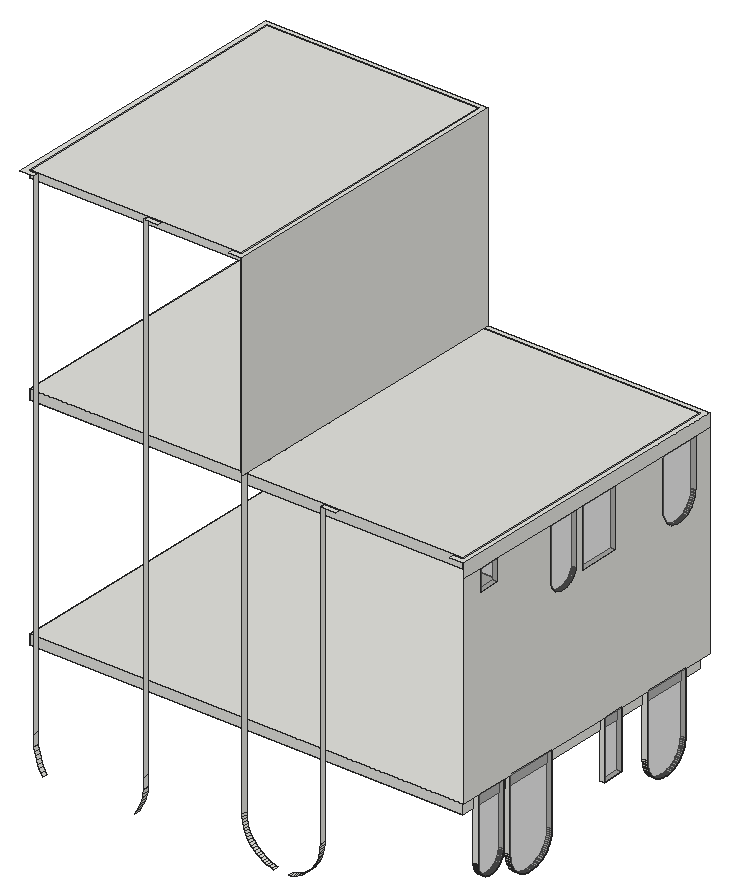
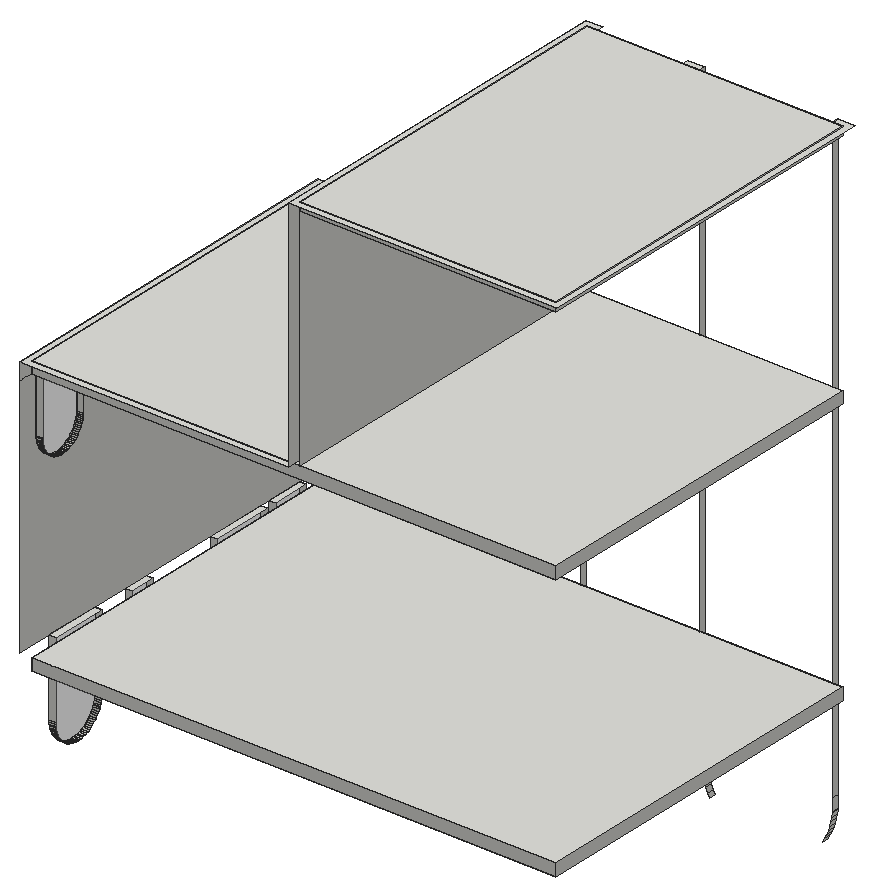
# SketchUp Ruby script. Lengths in inches.
U = 1.inch
M = Sketchup.active_model
def pt(a) = Geom::Point3d.new(a.map { |v| v * U })
def face(e, loops, mat)
  f = e.add_face(loops[0].map { |a| pt(a) })
  loops[1..].each { |l| e.add_face(l.map { |a| pt(a) }).erase! }
  f.material = f.back_material = mat if mat
  f
end
# faces: each face lists its corners as indices into pts; further lists are holes
def faces(e, pts, list, mat = nil) = list.each { |f| face(e, (f[0].is_a?(Array) ? f : [f]).map { |l| l.map { |i| pts[i] } }, mat) }
# xy, xz, yz: faces in a plane at the given z, y or x. An outline is a flat list of corners, or four numbers for a rectangle; further outlines are holes
def ring(l) = l.size == 4 ? [[l[0], l[1]], [l[2], l[1]], [l[2], l[3]], [l[0], l[3]]] : l.each_slice(2).to_a
def flat(e, list, mat, &to3) = list.each { |f| face(e, (f[0].is_a?(Array) ? f : [f]).map { |l| ring(l).map { |u, v| to3.(u, v) } }, mat) }
def xy(e, z, list, mat = nil) = flat(e, list, mat) { |x, y| [x, y, z] }
def xz(e, y, list, mat = nil) = flat(e, list, mat) { |x, z| [x, y, z] }
def yz(e, x, list, mat = nil) = flat(e, list, mat) { |y, z| [x, y, z] }
def lines(e, pts, list) = list.each { |a, b| e.add_line(pt(pts[a]), pt(pts[b])) }
# prism: a flat outline (further loops are holes) pulled along v
def prism(e, loops, v, mat = nil)
  f = face(e, loops, mat); d = Geom::Vector3d.new(v.map { |x| x * U })
  f.pushpull(f.normal.samedirection?(d) ? d.length : -d.length)
end
def box(e, o, s, mat = nil) = prism(e, [[o, [o[0] + s[0], o[1], o[2]], [o[0] + s[0], o[1] + s[1], o[2]], [o[0], o[1] + s[1], o[2]]]], [0, 0, s[2]], mat)
def at(x, y, z, deg = 0) = Geom::Transformation.translation(pt([x, y, z])) * Geom::Transformation.rotation(ORIGIN, Z_AXIS, deg.degrees)
def axes(o, x, y, z) = Geom::Transformation.new([*x, 0, *y, 0, *z, 0, *pt(o).to_a, 1])
def part(name) = M.definitions.add(name)
# library, detail: a bought-in or finely detailed component or shape, given as its bounding box
def library(name, o, s) = part(name).tap { |d| box(d.entities, o, s) }
def detail(e, o, s) = box(e.add_group.entities, o, s)
def put(e, d, t, mat = nil) = e.add_instance(d, t).tap { |i| i.material = mat if mat }
def group(e, t, mat = nil) = e.add_group.tap { |g| g.transformation = t; g.material = mat if mat }.entities
root = M.entities
M.materials.add("[Translucent Glass Gray]").color = [128, 128, 128]
M.materials["[Translucent Glass Gray]"].alpha = 0.5
c1 = part("Group\#2")
box(c1.entities,[0,0,0],[753.47,516,17])
box(root,[1479.625,496.08,1382],[368.1,516,12])
xy(root,576.55,[[2233.1,793.72,2242.1,831.72]])
xy(root,678.55,[[2233.1,518.83,2242.1,573.83],[2233.1,588.16,2242.1,679.32],[2233.1,793.72,2242.1,831.72],[2233.1,886.32,2242.1,969.32]])
xy(root,928.39,[[2233.1,745.0625,2242.1,818.41]])
xy(root,991.35,[[2233.1,523.83,2242.1,561.87]])
xy(root,1029.2,[[2233.1,523.83,2242.1,561.87],[2233.1,675.625,2242.1,733.55],[2233.1,745.0625,2242.1,818.41],[2233.1,919.74,2242.1,992.74]])
xy(root,1054,[[2218.1,487.08,2242.1,487.08,2242.1,1021.08,1856.72,1021.08,1856.72,1012.08,2233.1,1012.08,2233.1,496.08,2218.1,496.08],[1992.57,487.08,2019.16,496.08],[1847.72,496.08,1856.72,1012.08]])
xy(root,1394,[[1470.625,487.08,1494.625,487.08,1494.625,496.08,1479.625,496.08,1479.625,1012.08,1847.72,1012.08,1847.72,496.08,1832.72,496.08,1832.72,487.08,1856.72,487.08,1856.72,1021.08,1470.625,1021.08],[1685.42,487.08,1709.42,496.08]])
xz(root,487.08,[[1494.625,505.5,1494.625,523.51,1494.22,517.14,1494.25,510.75],[1685.42,505.5,1685.79,510.75,1685.82,517.14,1685.42,523.51]])
xz(root,518.83,[[2233.1,569.55,2242.1,678.55]])
xz(root,523.83,[[2233.1,991.35,2242.1,1029.2]])
xz(root,561.87,[[2233.1,991.35,2242.1,1029.2]])
xz(root,573.83,[[2233.1,569.55,2242.1,678.55]])
xz(root,588.16,[[2233.1,554.92,2242.1,678.55]])
xz(root,675.625,[[2233.1,938.71,2242.1,1029.2]])
xz(root,679.32,[[2233.1,554.92,2242.1,678.55]])
xz(root,733.55,[[2233.1,938.71,2242.1,1029.2]])
xz(root,745.0625,[[2233.1,928.39,2242.1,1029.2]])
xz(root,793.72,[[2233.1,576.55,2242.1,678.55]])
xz(root,818.41,[[2233.1,928.39,2242.1,1029.2]])
xz(root,831.72,[[2233.1,576.55,2242.1,678.55]])
xz(root,886.32,[[2233.1,569.55,2242.1,678.55]])
xz(root,919.74,[[2233.1,946.2,2242.1,1029.2]])
xz(root,969.32,[[2233.1,569.55,2242.1,678.55]])
xz(root,992.74,[[2233.1,946.2,2242.1,1029.2]])
yz(root,1494.625,[[487.08,505.5,496.08,523.51],[487.08,523.51,496.08,1394]])
yz(root,1685.42,[[487.08,505.5,496.08,523.51],[487.08,523.51,496.08,1394]])
yz(root,1847.72,[[496.08,1054,1012.08,1394]])
yz(root,1856.72,[[487.08,527,496.08,1054],[487.08,1054,1021.08,1394]])
yz(root,1992.57,[[487.08,527,496.08,1054]])
yz(root,2242.1,[[487.08,678.55,1021.08,678.55,1021.08,1029.2,992.74,1029.2,992.74,946.2,992.67,943.9,992.46,941.62,992.1,939.36,991.6,937.12,990.96,934.92,990.18,932.76,989.27,930.66,988.23,928.61,987.0625,926.64,985.77,924.74,984.37,922.93,982.85,921.21,981.23,919.59,979.51,918.07,977.7,916.67,975.8,915.38,973.83,914.21,971.78,913.17,969.68,912.26,967.52,911.48,965.32,910.84,963.08,910.34,960.82,909.98,958.54,909.77,956.24,909.7,953.95,909.77,951.67,909.98,949.4,910.34,947.17,910.84,944.96,911.48,942.81,912.26,940.7,913.17,938.66,914.21,936.6875,915.38,934.79,916.67,932.98,918.07,931.26,919.59,929.64,921.21,928.12,922.93,926.71,924.74,925.43,926.64,924.26,928.61,923.22,930.66,922.31,932.76,921.53,934.92,920.89,937.12,920.39,939.36,920.03,941.62,919.82,943.9,919.74,946.2,919.74,1029.2,818.41,1029.2,818.41,928.39,745.0625,928.39,745.0625,1029.2,733.55,1029.2,733.55,938.71,733.14,937.17,732.65,935.66,732.08,934.17,731.43,932.72,730.7,931.3,729.9,929.92,729.03,928.59,728.08,927.31,727.07,926.08,726,924.9,724.86,923.79,723.67,922.73,722.42,921.75,721.12,920.83,719.77,919.98,718.375,919.2,716.95,918.5,715.48,917.88,713.98,917.34,712.46,916.875,710.91,916.5,709.35,916.2,707.77,915.99,706.18,915.86,704.59,915.82,703,915.86,701.41,915.99,699.83,916.2,698.27,916.5,696.72,916.875,695.19,917.34,693.7,917.88,692.23,918.5,690.8,919.2,689.41,919.98,688.0625,920.83,686.76,921.75,685.51,922.73,684.32,923.79,683.18,924.9,682.1,926.08,681.09,927.31,680.15,928.59,679.28,929.92,678.47,931.3,677.75,932.72,677.1,934.17,676.53,935.66,676.04,937.17,675.625,938.71,675.625,1029.2,561.87,1029.2,561.87,991.35,523.83,991.35,523.83,1029.2,487.08,1029.2],[487.08,1029.2,1021.08,1054]])
yz(root,2242.1,[[633.74,509.34,636.6,509.43,639.45,509.7,642.28,510.15,645.07,510.78,647.82,511.57,650.51,512.54,653.14,513.68,655.69,514.98,658.16,516.4375,660.53,518.05,662.79,519.8,664.9375,521.7,666.96,523.72,668.86,525.87,670.61,528.13,672.22,530.5,673.68,532.96,674.98,535.52,676.11,538.14,677.08,540.84,677.88,543.59,678.51,546.38,678.96,549.21,679.23,552.0625,679.32,554.92,679.32,678.55,588.16,678.55,588.16,554.92,588.25,552.0625,588.52,549.21,588.96,546.38,589.59,543.59,590.39,540.84,591.36,538.14,592.49,535.52,593.79,532.96,595.25,530.5,596.86,528.13,598.62,525.87,600.51,523.72,602.53,521.7,604.68,519.8,606.94,518.05,609.3125,516.4375,611.78,514.98,614.33,513.68,616.96,512.54,619.65,511.57,622.4,510.78,625.19,510.15,628.02,509.7,630.875,509.43],[927.82,528.05,930.42,528.14,933.02,528.38,935.59,528.79,938.14,529.36,940.64,530.09,943.09,530.97,945.49,532,947.81,533.1875,950.05,534.51,952.21,535.98,954.27,537.58,956.22,539.3,958.07,541.15,959.79,543.1,961.39,545.16,962.86,547.32,964.18,549.5625,965.37,551.88,966.4,554.28,966.63,554.92,967.28,556.73,968.01,559.23,968.58,561.78,968.99,564.35,969.23,566.95,969.32,569.55,969.32,678.55,886.32,678.55,886.32,569.55,886.4,566.95,886.64,564.35,887.05,561.78,887.62,559.23,888.35,556.73,889,554.92,889.23,554.28,890.27,551.88,891.45,549.5625,892.78,547.32,894.24,545.16,895.84,543.1,897.5625,541.15,899.41,539.3,901.36,537.58,903.42,535.98,905.58,534.51,907.82,533.1875,910.15,532,912.54,530.97,914.99,530.09,917.5,529.36,920.04,528.79,922.61,528.38,925.21,528.14],[546.33,542.05,548.05,542.11,549.77,542.27,551.48,542.54,553.17,542.92,554.82,543.4,556.45,543.99,558.04,544.67,559.58,545.46,561.0625,546.33,562.49,547.31,563.86,548.36,565.15,549.51,566.375,550.73,567.52,552.02,568.57,553.39,569.55,554.82,569.61,554.92,570.43,556.31,571.21,557.84,571.9,559.43,572.48,561.06,572.96,562.71,573.34,564.4,573.61,566.11,573.77,567.83,573.83,569.55,573.83,678.55,518.83,678.55,518.83,569.55,518.88,567.83,519.04,566.11,519.3125,564.4,519.69,562.71,520.17,561.06,520.76,559.43,521.44,557.84,522.23,556.31,523.05,554.92,523.11,554.82,524.08,553.39,525.14,552.02,526.28,550.73,527.5,549.51,528.8,548.36,530.16,547.31,531.59,546.33,533.08,545.46,534.62,544.67,536.2,543.99,537.83,543.4,539.49,542.92,541.17,542.54,542.88,542.27,544.6,542.11],[793.72,576.55,831.72,678.55],[956.24,909.7,958.54,909.77,960.82,909.98,963.08,910.34,965.32,910.84,967.52,911.48,969.68,912.26,971.78,913.17,973.83,914.21,975.8,915.38,977.7,916.67,979.51,918.07,981.23,919.59,982.85,921.21,984.37,922.93,985.77,924.74,987.0625,926.64,988.23,928.61,989.27,930.66,990.18,932.76,990.96,934.92,991.6,937.12,992.1,939.36,992.46,941.62,992.67,943.9,992.74,946.2,992.74,1029.2,919.74,1029.2,919.74,946.2,919.82,943.9,920.03,941.62,920.39,939.36,920.89,937.12,921.53,934.92,922.31,932.76,923.22,930.66,924.26,928.61,925.43,926.64,926.71,924.74,928.12,922.93,929.64,921.21,931.26,919.59,932.98,918.07,934.79,916.67,936.6875,915.38,938.66,914.21,940.7,913.17,942.81,912.26,944.96,911.48,947.17,910.84,949.4,910.34,951.67,909.98,953.95,909.77],
  [704.59,915.82,706.18,915.86,707.77,915.99,709.35,916.2,710.91,916.5,712.46,916.875,713.98,917.34,715.48,917.88,716.95,918.5,718.375,919.2,719.77,919.98,721.12,920.83,722.42,921.75,723.67,922.73,724.86,923.79,726,924.9,727.07,926.08,728.08,927.31,729.03,928.59,729.9,929.92,730.7,931.3,731.43,932.72,732.08,934.17,732.65,935.66,733.14,937.17,733.55,938.71,733.55,1029.2,675.625,1029.2,675.625,938.71,676.04,937.17,676.53,935.66,677.1,934.17,677.75,932.72,678.47,931.3,679.28,929.92,680.15,928.59,681.09,927.31,682.1,926.08,683.18,924.9,684.32,923.79,685.51,922.73,686.76,921.75,688.0625,920.83,689.41,919.98,690.8,919.2,692.23,918.5,693.7,917.88,695.19,917.34,696.72,916.875,698.27,916.5,699.83,916.2,701.41,915.99,703,915.86],[745.0625,928.39,818.41,1029.2],[523.83,991.35,561.87,1029.2]],"[Translucent Glass Gray]")
p = [[1907.75,487.08,461.21],[1911.92,487.08,460.27],[1911.92,496.08,460.27],[1907.75,496.08,461.21],[1937.37,487.08,460.27],[1941.54,487.08,461.21],
  [1941.54,496.08,461.21],[1937.37,496.08,460.27],[1903.65,487.08,462.4],[1903.65,496.08,462.4],[1945.64,487.08,462.4],[1945.64,496.08,462.4],
  [1899.64,487.08,463.84],[1899.64,496.08,463.84],[1949.65,487.08,463.84],[1949.65,496.08,463.84],[1506.11,487.08,468.05],[1509.38,487.08,462.5625],
  [1509.38,496.08,462.5625],[1506.11,496.08,468.05],[1670.66,487.08,462.5625],[1673.93,487.08,468.05],[1673.93,496.08,468.05],[1670.66,496.08,462.5625],
  [1895.72,487.08,465.54],[1895.72,496.08,465.54],[1953.57,487.08,465.54],[1953.57,496.08,465.54],[1891.92,487.08,467.47],[1891.92,496.08,467.47],
  [1957.37,487.08,467.47],[1957.37,496.08,467.47],[1957.125,496.08,467.35],[1888.25,487.08,469.65],[1888.25,496.08,469.65],[1961.04,487.08,469.65],
  [1961.04,496.08,469.65],[1503.21,487.08,473.74],[1503.21,496.08,473.74],[1676.83,487.08,473.74],[1676.83,496.08,473.74],[1884.72,487.08,472.04],
  [1884.72,496.08,472.04],[1964.57,487.08,472.04],[1964.57,496.08,472.04],[1881.35,487.08,474.66],[1881.35,496.08,474.66],[1967.94,487.08,474.66],
  [1967.94,496.08,474.66],[1500.7,487.08,479.62],[1500.7,496.08,479.62],[1679.34,487.08,479.62],[1679.34,496.08,479.62],[1878.14,487.08,477.48],
  [1878.14,496.08,477.48],[1971.14,487.08,477.48],[1971.14,496.08,477.48],[1875.125,487.08,480.5],[1875.125,496.08,480.5],[1974.16,487.08,480.5],
  [1974.16,496.08,480.5],[1498.58,487.08,485.64],[1498.58,496.08,485.64],[1681.46,487.08,485.64],[1681.46,496.08,485.64],[1872.3,487.08,483.7],
  [1872.3,496.08,483.7],[1976.98,487.08,483.7],[1976.98,496.08,483.7],[1869.6875,487.08,487.07],[1869.6875,496.08,487.07],[1979.6,487.08,487.07],
  [1979.6,496.08,487.07],[1496.875,487.08,491.8],[1496.875,496.08,491.8],[1683.17,487.08,491.8],[1683.17,496.08,491.8],[1867.29,487.08,490.6],
  [1867.29,496.08,490.6],[1982,487.08,490.6],[1982,496.08,490.6],[1865.12,487.08,494.28],[1865.12,496.08,494.28],[1984.17,487.08,494.28],
  [1984.17,496.08,494.28],[1495.58,487.08,498.05],[1495.58,496.08,498.05],[1684.46,487.08,498.05],[1684.46,496.08,498.05],[1863.18,487.08,498.08],
  [1863.18,496.08,498.08],[1986.11,487.08,498.08],[1986.11,496.08,498.08],[1494.7,487.08,504.38],[1494.7,496.08,504.38],[1685.34,487.08,504.38],
  [1685.34,496.08,504.38],[1861.49,487.08,501.99],[1861.49,496.08,501.99],[1987.8,487.08,501.99],[1987.8,496.08,501.99],[1860.04,487.08,506.01],
  [1860.04,496.08,506.01],[1989.25,487.08,506.01],[1989.25,496.08,506.01],[1494.625,487.08,505.5],[1494.625,496.08,505.5],[1685.42,487.08,505.5],
  [1685.42,496.08,505.5],[1858.85,487.08,510.11],[1858.85,496.08,510.11],[1990.4375,487.08,510.11],[1990.4375,496.08,510.11],[2242.1,630.875,509.43],
  [2242.1,633.74,509.34],[2233.1,633.74,509.34],[2233.1,630.875,509.43],[2242.1,636.6,509.43],[2233.1,636.6,509.43],[2242.1,628.02,509.7],
  [2233.1,628.02,509.7],[2242.1,639.45,509.7],[2233.1,639.45,509.7],[2242.1,625.19,510.15],[2233.1,625.19,510.15],[2242.1,642.28,510.15],
  [2233.1,642.28,510.15],[1857.92,487.08,514.27],[1857.92,496.08,514.27],[1991.37,487.08,514.27],[1991.37,496.08,514.27],[2242.1,622.4,510.78],
  [2233.1,622.4,510.78],[2242.1,645.07,510.78],[2233.1,645.07,510.78],[2242.1,619.65,511.57],[2233.1,619.65,511.57],[2242.1,647.82,511.57],
  [2233.1,647.82,511.57],[2242.1,616.96,512.54],[2233.1,616.96,512.54],[2242.1,650.51,512.54],[2233.1,650.51,512.54],[2242.1,614.33,513.68],
  [2233.1,614.33,513.68],[2242.1,653.14,513.68],[2233.1,653.14,513.68],[2242.1,611.78,514.98],[2233.1,611.78,514.98],[2242.1,655.69,514.98],
  [2233.1,655.69,514.98],[1857.25,487.08,518.49],[1857.25,496.08,518.49],[1992.04,487.08,518.49],[1992.04,496.08,518.49],[2242.1,609.3125,516.4375],
  [2233.1,609.3125,516.4375],[2242.1,658.16,516.4375],[2233.1,658.16,516.4375],[2242.1,606.94,518.05],[2233.1,606.94,518.05],[2242.1,660.53,518.05],
  [2233.1,660.53,518.05],[2242.1,604.68,519.8],[2233.1,604.68,519.8],[2242.1,662.79,519.8],[2233.1,662.79,519.8],[1856.85,487.08,522.73],
  [1856.85,496.08,522.73],[1992.4375,487.08,522.73],[1992.4375,496.08,522.73],[2242.1,602.53,521.7],[2233.1,602.53,521.7],[2242.1,664.9375,521.7],
  [2233.1,664.9375,521.7],[2242.1,600.51,523.72],[2233.1,600.51,523.72],[2242.1,666.96,523.72],[2233.1,666.96,523.72],[1856.72,487.08,527],
  [1856.72,496.08,527],[1992.57,487.08,527],[1992.57,496.08,527],[2242.1,598.62,525.87],[2233.1,598.62,525.87],[2242.1,668.86,525.87],
  [2233.1,668.86,525.87],[2242.1,596.86,528.13],[2233.1,596.86,528.13],[2242.1,670.61,528.13],[2233.1,670.61,528.13],[2242.1,595.25,530.5],
  [2233.1,595.25,530.5],[2242.1,672.22,530.5],[2233.1,672.22,530.5],[2242.1,922.61,528.38],[2242.1,925.21,528.14],[2233.1,925.21,528.14],
  [2233.1,922.61,528.38],[2242.1,927.82,528.05],[2233.1,927.82,528.05],[2242.1,930.42,528.14],[2233.1,930.42,528.14],[2242.1,933.02,528.38],
  [2233.1,933.02,528.38],[2242.1,920.04,528.79],[2233.1,920.04,528.79],[2242.1,935.59,528.79],[2233.1,935.59,528.79],[2242.1,917.5,529.36],
  [2233.1,917.5,529.36],[2242.1,938.14,529.36],[2233.1,938.14,529.36],[2242.1,914.99,530.09],[2233.1,914.99,530.09],[2242.1,940.64,530.09],
  [2233.1,940.64,530.09],[2242.1,912.54,530.97],[2233.1,912.54,530.97],[2242.1,943.09,530.97],[2233.1,943.09,530.97],[2242.1,593.79,532.96],
  [2233.1,593.79,532.96],[2242.1,673.68,532.96],[2233.1,673.68,532.96],[2242.1,910.15,532],[2233.1,910.15,532],[2242.1,945.49,532],
  [2233.1,945.49,532],[2242.1,907.82,533.1875],[2233.1,907.82,533.1875],[2242.1,947.81,533.1875],[2233.1,947.81,533.1875],[2242.1,592.49,535.52],
  [2233.1,592.49,535.52],[2242.1,674.98,535.52],[2233.1,674.98,535.52],[2242.1,905.58,534.51],[2233.1,905.58,534.51],[2242.1,950.05,534.51],
  [2233.1,950.05,534.51],[2242.1,903.42,535.98],[2233.1,903.42,535.98],[2242.1,952.21,535.98],[2233.1,952.21,535.98],[2242.1,591.36,538.14],
  [2233.1,591.36,538.14],[2242.1,676.11,538.14],[2233.1,676.11,538.14],[2242.1,901.36,537.58],[2233.1,901.36,537.58],[2242.1,954.27,537.58],
  [2233.1,954.27,537.58],[2242.1,899.41,539.3],[2233.1,899.41,539.3],[2242.1,956.22,539.3],[2233.1,956.22,539.3],[2242.1,590.39,540.84],
  [2233.1,590.39,540.84],[2242.1,677.08,540.84],[2233.1,677.08,540.84],[2242.1,897.5625,541.15],[2233.1,897.5625,541.15],[2242.1,958.07,541.15],
  [2233.1,958.07,541.15],[2242.1,589.59,543.59],[2233.1,589.59,543.59],[2242.1,677.88,543.59],[2233.1,677.88,543.59],[2242.1,895.84,543.1],
  [2233.1,895.84,543.1],[2242.1,959.79,543.1],[2233.1,959.79,543.1],[2242.1,542.88,542.27],[2242.1,544.6,542.11],[2233.1,544.6,542.11],
  [2233.1,542.88,542.27],[2242.1,546.33,542.05],[2233.1,546.33,542.05],[2242.1,548.05,542.11],[2233.1,548.05,542.11],[2242.1,549.77,542.27],
  [2233.1,549.77,542.27],[2242.1,541.17,542.54],[2233.1,541.17,542.54],[2242.1,551.48,542.54],[2233.1,551.48,542.54],[2242.1,539.49,542.92],
  [2233.1,539.49,542.92],[2242.1,553.17,542.92],[2233.1,553.17,542.92],[2242.1,537.83,543.4],[2233.1,537.83,543.4],[2242.1,554.82,543.4],
  [2233.1,554.82,543.4],[2242.1,894.24,545.16],[2233.1,894.24,545.16],[2242.1,961.39,545.16],[2233.1,961.39,545.16],[2242.1,536.2,543.99],
  [2233.1,536.2,543.99],[2242.1,556.45,543.99],[2233.1,556.45,543.99],[2242.1,588.96,546.38],[2233.1,588.96,546.38],[2242.1,678.51,546.38],
  [2233.1,678.51,546.38],[2242.1,534.62,544.67],[2233.1,534.62,544.67],[2242.1,558.04,544.67],[2233.1,558.04,544.67],[2242.1,533.08,545.46],
  [2233.1,533.08,545.46],[2242.1,559.58,545.46],[2233.1,559.58,545.46],[2242.1,892.78,547.32],[2233.1,892.78,547.32],[2242.1,962.86,547.32],
  [2233.1,962.86,547.32],[2242.1,531.59,546.33],[2233.1,531.59,546.33],[2242.1,561.0625,546.33],[2233.1,561.0625,546.33],[2242.1,530.16,547.31],
  [2233.1,530.16,547.31],[2242.1,562.49,547.31],[2233.1,562.49,547.31],[2242.1,588.52,549.21],[2233.1,588.52,549.21],[2242.1,678.96,549.21],
  [2233.1,678.96,549.21],[2242.1,528.8,548.36],[2233.1,528.8,548.36],[2242.1,563.86,548.36],[2233.1,563.86,548.36],[2242.1,891.45,549.5625],
  [2233.1,891.45,549.5625],[2242.1,964.18,549.5625],[2233.1,964.18,549.5625],[2242.1,527.5,549.51],[2233.1,527.5,549.51],[2242.1,565.15,549.51],
  [2233.1,565.15,549.51],[2242.1,588.25,552.0625],[2233.1,588.25,552.0625],[2242.1,679.23,552.0625],[2233.1,679.23,552.0625],[2242.1,526.28,550.73],
  [2233.1,526.28,550.73],[2242.1,566.375,550.73],[2233.1,566.375,550.73],[2242.1,890.27,551.88],[2233.1,890.27,551.88],[2242.1,965.37,551.88],
  [2233.1,965.37,551.88],[2242.1,525.14,552.02],[2233.1,525.14,552.02],[2242.1,567.52,552.02],[2233.1,567.52,552.02],[2242.1,889.23,554.28],
  [2233.1,889.23,554.28],[2242.1,966.4,554.28],[2233.1,966.4,554.28],[2242.1,524.08,553.39],[2233.1,524.08,553.39],[2242.1,568.57,553.39],
  [2233.1,568.57,553.39],[2242.1,588.16,554.92],[2233.1,588.16,554.92],[2242.1,679.32,554.92],[2233.1,679.32,554.92],[2242.1,523.11,554.82],
  [2233.1,523.11,554.82],[2242.1,569.55,554.82],[2233.1,569.55,554.82],[2242.1,889,554.92],[2233.1,889,554.92],[2242.1,966.63,554.92],
  [2233.1,966.63,554.92],[2242.1,523.05,554.92],[2233.1,523.05,554.92],[2242.1,569.61,554.92],[2233.1,569.61,554.92],[2242.1,522.23,556.31],
  [2233.1,522.23,556.31],[2242.1,570.43,556.31],[2233.1,570.43,556.31],[2242.1,888.35,556.73],[2233.1,888.35,556.73],[2242.1,967.28,556.73],
  [2233.1,967.28,556.73],[2242.1,521.44,557.84],[2233.1,521.44,557.84],[2242.1,571.21,557.84],[2233.1,571.21,557.84],[2242.1,887.62,559.23],
  [2233.1,887.62,559.23],[2242.1,968.01,559.23],[2233.1,968.01,559.23],[2242.1,520.76,559.43],[2233.1,520.76,559.43],[2242.1,571.9,559.43],
  [2233.1,571.9,559.43],[2242.1,887.05,561.78],[2233.1,887.05,561.78],[2242.1,968.58,561.78],[2233.1,968.58,561.78],[2242.1,520.17,561.06],
  [2233.1,520.17,561.06],[2242.1,572.48,561.06],[2233.1,572.48,561.06],[2242.1,519.69,562.71],[2233.1,519.69,562.71],[2242.1,572.96,562.71],
  [2233.1,572.96,562.71],[2242.1,886.64,564.35],[2233.1,886.64,564.35],[2242.1,968.99,564.35],[2233.1,968.99,564.35],[2242.1,519.3125,564.4],
  [2233.1,519.3125,564.4],[2242.1,573.34,564.4],[2233.1,573.34,564.4],[2242.1,519.04,566.11],[2233.1,519.04,566.11],[2242.1,573.61,566.11],
  [2233.1,573.61,566.11],[2242.1,886.4,566.95],[2233.1,886.4,566.95],[2242.1,969.23,566.95],[2233.1,969.23,566.95],[2242.1,518.88,567.83],
  [2233.1,518.88,567.83],[2242.1,573.77,567.83],[2233.1,573.77,567.83],[2242.1,886.32,569.55],[2233.1,886.32,569.55],[2242.1,969.32,569.55],
  [2233.1,969.32,569.55],[2242.1,518.83,569.55],[2233.1,518.83,569.55],[2242.1,573.83,569.55],[2233.1,573.83,569.55],[2242.1,953.95,909.77],
  [2242.1,956.24,909.7],[2233.1,956.24,909.7],[2233.1,953.95,909.77],[2242.1,958.54,909.77],[2233.1,958.54,909.77],[2242.1,951.67,909.98],
  [2233.1,951.67,909.98],[2242.1,960.82,909.98],[2233.1,960.82,909.98],[2242.1,949.4,910.34],[2233.1,949.4,910.34],[2242.1,963.08,910.34],
  [2233.1,963.08,910.34],[2242.1,947.17,910.84],[2233.1,947.17,910.84],[2242.1,965.32,910.84],[2233.1,965.32,910.84],[2242.1,944.96,911.48],
  [2233.1,944.96,911.48],[2242.1,967.52,911.48],[2233.1,967.52,911.48],[2242.1,942.81,912.26],[2233.1,942.81,912.26],[2242.1,969.68,912.26],
  [2233.1,969.68,912.26],[2242.1,940.7,913.17],[2233.1,940.7,913.17],[2242.1,971.78,913.17],[2233.1,971.78,913.17],[2242.1,938.66,914.21],
  [2233.1,938.66,914.21],[2242.1,973.83,914.21],[2233.1,973.83,914.21],[2242.1,936.6875,915.38],[2233.1,936.6875,915.38],[2242.1,975.8,915.38],
  [2233.1,975.8,915.38],[2242.1,934.79,916.67],[2233.1,934.79,916.67],[2242.1,977.7,916.67],[2233.1,977.7,916.67],[2242.1,703,915.86],
  [2242.1,704.59,915.82],[2233.1,704.59,915.82],[2233.1,703,915.86],[2242.1,706.18,915.86],[2233.1,706.18,915.86],[2242.1,701.41,915.99],
  [2233.1,701.41,915.99],[2242.1,707.77,915.99],[2233.1,707.77,915.99],[2242.1,699.83,916.2],[2233.1,699.83,916.2],[2242.1,709.35,916.2],
  [2233.1,709.35,916.2],[2242.1,698.27,916.5],[2233.1,698.27,916.5],[2242.1,710.91,916.5],[2233.1,710.91,916.5],[2242.1,696.72,916.875],
  [2233.1,696.72,916.875],[2242.1,712.46,916.875],[2233.1,712.46,916.875],[2242.1,932.98,918.07],[2233.1,932.98,918.07],[2242.1,979.51,918.07],
  [2233.1,979.51,918.07],[2242.1,695.19,917.34],[2233.1,695.19,917.34],[2242.1,713.98,917.34],[2233.1,713.98,917.34],[2242.1,693.7,917.88],
  [2233.1,693.7,917.88],[2242.1,715.48,917.88],[2233.1,715.48,917.88],[2242.1,692.23,918.5],[2233.1,692.23,918.5],[2242.1,716.95,918.5],
  [2233.1,716.95,918.5],[2242.1,931.26,919.59],[2233.1,931.26,919.59],[2242.1,981.23,919.59],[2233.1,981.23,919.59],[2242.1,690.8,919.2],
  [2233.1,690.8,919.2],[2242.1,718.375,919.2],[2233.1,718.375,919.2],[2242.1,689.41,919.98],[2233.1,689.41,919.98],[2242.1,719.77,919.98],
  [2233.1,719.77,919.98],[2242.1,929.64,921.21],[2233.1,929.64,921.21],[2242.1,982.85,921.21],[2233.1,982.85,921.21],[2242.1,688.0625,920.83],
  [2233.1,688.0625,920.83],[2242.1,721.12,920.83],[2233.1,721.12,920.83],[2242.1,686.76,921.75],[2233.1,686.76,921.75],[2242.1,722.42,921.75],
  [2233.1,722.42,921.75],[2242.1,928.12,922.93],[2233.1,928.12,922.93],[2242.1,984.37,922.93],[2233.1,984.37,922.93],[2242.1,685.51,922.73],
  [2233.1,685.51,922.73],[2242.1,723.67,922.73],[2233.1,723.67,922.73],[2242.1,684.32,923.79],[2233.1,684.32,923.79],[2242.1,724.86,923.79],
  [2233.1,724.86,923.79],[2242.1,926.71,924.74],[2233.1,926.71,924.74],[2242.1,985.77,924.74],[2233.1,985.77,924.74],[2242.1,683.18,924.9],
  [2233.1,683.18,924.9],[2242.1,726,924.9],[2233.1,726,924.9],[2242.1,925.43,926.64],[2233.1,925.43,926.64],[2242.1,987.0625,926.64],
  [2233.1,987.0625,926.64],[2242.1,682.1,926.08],[2233.1,682.1,926.08],[2242.1,727.07,926.08],[2233.1,727.07,926.08],[2242.1,681.09,927.31],
  [2233.1,681.09,927.31],[2242.1,728.08,927.31],[2233.1,728.08,927.31],[2242.1,924.26,928.61],[2233.1,924.26,928.61],[2242.1,988.23,928.61],
  [2233.1,988.23,928.61],[2242.1,680.15,928.59],[2233.1,680.15,928.59],[2242.1,729.03,928.59],[2233.1,729.03,928.59],[2242.1,679.28,929.92],
  [2233.1,679.28,929.92],[2242.1,729.9,929.92],[2233.1,729.9,929.92],[2242.1,923.22,930.66],[2233.1,923.22,930.66],[2242.1,989.27,930.66],
  [2233.1,989.27,930.66],[2242.1,678.47,931.3],[2233.1,678.47,931.3],[2242.1,730.7,931.3],[2233.1,730.7,931.3],[2242.1,922.31,932.76],
  [2233.1,922.31,932.76],[2242.1,990.18,932.76],[2233.1,990.18,932.76],[2242.1,677.75,932.72],[2233.1,677.75,932.72],[2242.1,731.43,932.72],
  [2233.1,731.43,932.72],[2242.1,677.1,934.17],[2233.1,677.1,934.17],[2242.1,732.08,934.17],[2233.1,732.08,934.17],[2242.1,921.53,934.92],
  [2233.1,921.53,934.92],[2242.1,990.96,934.92],[2233.1,990.96,934.92],[2242.1,676.53,935.66],[2233.1,676.53,935.66],[2242.1,732.65,935.66],
  [2233.1,732.65,935.66],[2242.1,920.89,937.12],[2233.1,920.89,937.12],[2242.1,991.6,937.12],[2233.1,991.6,937.12],[2242.1,676.04,937.17],
  [2233.1,676.04,937.17],[2242.1,733.14,937.17],[2233.1,733.14,937.17],[2242.1,920.39,939.36],[2233.1,920.39,939.36],[2242.1,992.1,939.36],
  [2233.1,992.1,939.36],[2242.1,675.625,938.71],[2233.1,675.625,938.71],[2242.1,733.55,938.71],[2233.1,733.55,938.71],[2242.1,920.03,941.62],
  [2233.1,920.03,941.62],[2242.1,992.46,941.62],[2233.1,992.46,941.62],[2242.1,919.82,943.9],[2233.1,919.82,943.9],[2242.1,992.67,943.9],
  [2233.1,992.67,943.9],[2242.1,919.74,946.2],[2233.1,919.74,946.2],[2242.1,992.74,946.2],[2233.1,992.74,946.2]]
faces(root,p,[[0,1,2,3],[4,5,6,7],[8,0,3,9],[5,10,11,6],[12,8,9,13],[10,14,15,11],[16,17,18,19],[20,21,22,23],
  [24,12,13,25],[14,26,27,15],[28,24,25,29],[26,30,31,32,27],[33,28,29,34],[30,35,36,31],[37,16,19,38],[21,39,40,22],
  [41,33,34,42],[35,43,44,36],[45,41,42,46],[43,47,48,44],[49,37,38,50],[39,51,52,40],[53,45,46,54],[47,55,56,48],
  [57,53,54,58],[55,59,60,56],[61,49,50,62],[51,63,64,52],[65,57,58,66],[59,67,68,60],[69,65,66,70],[67,71,72,68],
  [73,61,62,74],[63,75,76,64],[77,69,70,78],[71,79,80,72],[81,77,78,82],[79,83,84,80],[85,73,74,86],[75,87,88,76],
  [89,81,82,90],[83,91,92,84],[93,85,86,94],[87,95,96,88],[97,89,90,98],[91,99,100,92],[101,97,98,102],[99,103,104,100],
  [105,93,94,106],[95,107,108,96],[109,101,102,110],[103,111,112,104],[113,114,115,116],[114,117,118,115],[119,113,116,120],[117,121,122,118],
  [123,119,120,124],[121,125,126,122],[127,109,110,128],[111,129,130,112],[131,123,124,132],[125,133,134,126],[135,131,132,136],[133,137,138,134],
  [139,135,136,140],[137,141,142,138],[143,139,140,144],[141,145,146,142],[147,143,144,148],[145,149,150,146],[151,127,128,152],[129,153,154,130],
  [155,147,148,156],[149,157,158,150],[159,155,156,160],[157,161,162,158],[163,159,160,164],[161,165,166,162],[167,151,152,168],[153,169,170,154],
  [171,163,164,172],[165,173,174,166],[175,171,172,176],[173,177,178,174],[179,167,168,180],[169,181,182,170],[183,175,176,184],[177,185,186,178],
  [187,183,184,188],[185,189,190,186],[191,187,188,192],[189,193,194,190],[195,196,197,198],[196,199,200,197],[199,201,202,200],[201,203,204,202],
  [205,195,198,206],[203,207,208,204],[209,205,206,210],[207,211,212,208],[213,209,210,214],[211,215,216,212],[217,213,214,218],[215,219,220,216],
  [221,191,192,222],[193,223,224,194],[225,217,218,226],[219,227,228,220],[229,225,226,230],[227,231,232,228],[233,221,222,234],[223,235,236,224],
  [237,229,230,238],[231,239,240,232],[241,237,238,242],[239,243,244,240],[245,233,234,246],[235,247,248,236],[249,241,242,250],[243,251,252,244],
  [253,249,250,254],[251,255,256,252],[257,245,246,258],[247,259,260,248],[261,253,254,262],[255,263,264,256],[265,257,258,266],[259,267,268,260],
  [269,261,262,270],[263,271,272,264],[273,274,275,276],[274,277,278,275],[277,279,280,278],[279,281,282,280],[283,273,276,284],[281,285,286,282],
  [287,283,284,288],[285,289,290,286],[291,287,288,292],[289,293,294,290],[295,269,270,296],[271,297,298,272],[299,291,292,300],[293,301,302,294],
  [303,265,266,304],[267,305,306,268],[307,299,300,308],[301,309,310,302],[311,307,308,312],[309,313,314,310],[315,295,296,316],[297,317,318,298],
  [319,311,312,320],[313,321,322,314],[323,319,320,324],[321,325,326,322],[327,303,304,328],[305,329,330,306],[331,323,324,332],[325,333,334,326],
  [335,315,316,336],[317,337,338,318],[339,331,332,340],[333,341,342,334],[343,327,328,344],[329,345,346,330],[347,339,340,348],[341,349,350,342],
  [351,335,336,352],[337,353,354,338],[355,347,348,356],[349,357,358,350],[359,351,352,360],[353,361,362,354],[363,355,356,364],[357,365,366,358],
  [367,343,344,368],[345,369,370,346],[371,363,364,372],[365,373,374,366],[375,359,360,376],[361,377,378,362],[379,371,372,380],[373,381,382,374],
  [383,379,380,384],[381,385,386,382],[387,375,376,388],[377,389,390,378],[391,383,384,392],[385,393,394,386],[395,387,388,396],[389,397,398,390],
  [399,391,392,400],[393,401,402,394],[403,395,396,404],[397,405,406,398],[407,399,400,408],[401,409,410,402],[411,407,408,412],[409,413,414,410],
  [415,403,404,416],[405,417,418,406],[419,411,412,420],[413,421,422,414],[423,419,420,424],[421,425,426,422],[427,415,416,428],[417,429,430,418],
  [431,423,424,432],[425,433,434,426],[435,427,428,436],[429,437,438,430],[439,431,432,440],[433,441,442,434],[443,444,445,446],[444,447,448,445],
  [449,443,446,450],[447,451,452,448],[453,449,450,454],[451,455,456,452],[457,453,454,458],[455,459,460,456],[461,457,458,462],[459,463,464,460],
  [465,461,462,466],[463,467,468,464],[469,465,466,470],[467,471,472,468],[473,469,470,474],[471,475,476,472],[477,473,474,478],[475,479,480,476],
  [481,477,478,482],[479,483,484,480],[485,486,487,488],[486,489,490,487],[491,485,488,492],[489,493,494,490],[495,491,492,496],[493,497,498,494],
  [499,495,496,500],[497,501,502,498],[503,499,500,504],[501,505,506,502],[507,481,482,508],[483,509,510,484],[511,503,504,512],[505,513,514,506],
  [515,511,512,516],[513,517,518,514],[519,515,516,520],[517,521,522,518],[523,507,508,524],[509,525,526,510],[527,519,520,528],[521,529,530,522],
  [531,527,528,532],[529,533,534,530],[535,523,524,536],[525,537,538,526],[539,531,532,540],[533,541,542,534],[543,539,540,544],[541,545,546,542],
  [547,535,536,548],[537,549,550,538],[551,543,544,552],[545,553,554,546],[555,551,552,556],[553,557,558,554],[559,547,548,560],[549,561,562,550],
  [563,555,556,564],[557,565,566,558],[567,559,560,568],[561,569,570,562],[571,563,564,572],[565,573,574,566],[575,571,572,576],[573,577,578,574],
  [579,567,568,580],[569,581,582,570],[583,575,576,584],[577,585,586,578],[587,583,584,588],[585,589,590,586],[591,579,580,592],[581,593,594,582],
  [595,587,588,596],[589,597,598,590],[599,591,592,600],[593,601,602,594],[603,595,596,604],[597,605,606,598],[607,603,604,608],[605,609,610,606],
  [611,599,600,612],[601,613,614,602],[615,607,608,616],[609,617,618,610],[619,611,612,620],[613,621,622,614],[623,615,616,624],[617,625,626,618],
  [627,619,620,628],[621,629,630,622],[631,623,624,632],[625,633,634,626],[635,627,628,636],[629,637,638,630],[639,635,636,640],[637,641,642,638],
  [643,639,640,644],[641,645,646,642]])
put(root,c1,at(1479.625,496.08,654.82))
put(root,c1,at(1479.625,496.08,1037))
